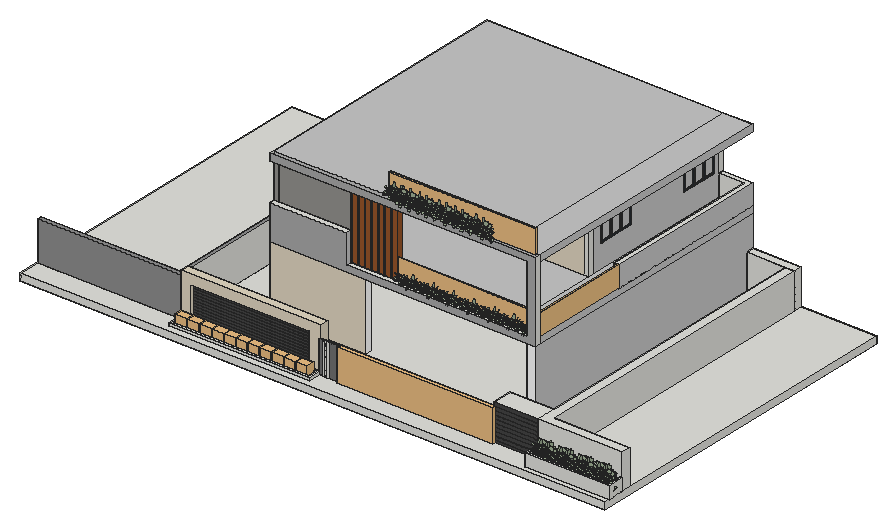
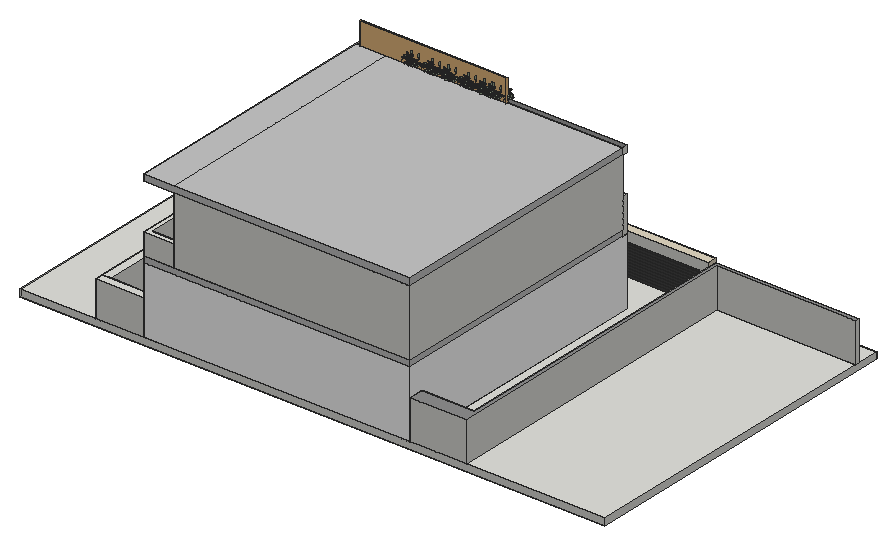
# SketchUp Ruby script. Lengths in inches.
U = 1.inch
M = Sketchup.active_model
def pt(a) = Geom::Point3d.new(a.map { |v| v * U })
def face(e, loops, mat)
  f = e.add_face(loops[0].map { |a| pt(a) })
  loops[1..].each { |l| e.add_face(l.map { |a| pt(a) }).erase! }
  f.material = f.back_material = mat if mat
  f
end
# faces: each face lists its corners as indices into pts; further lists are holes
def faces(e, pts, list, mat = nil) = list.each { |f| face(e, (f[0].is_a?(Array) ? f : [f]).map { |l| l.map { |i| pts[i] } }, mat) }
# xy, xz, yz: faces in a plane at the given z, y or x. An outline is a flat list of corners, or four numbers for a rectangle; further outlines are holes
def ring(l) = l.size == 4 ? [[l[0], l[1]], [l[2], l[1]], [l[2], l[3]], [l[0], l[3]]] : l.each_slice(2).to_a
def flat(e, list, mat, &to3) = list.each { |f| face(e, (f[0].is_a?(Array) ? f : [f]).map { |l| ring(l).map { |u, v| to3.(u, v) } }, mat) }
def xy(e, z, list, mat = nil) = flat(e, list, mat) { |x, y| [x, y, z] }
def xz(e, y, list, mat = nil) = flat(e, list, mat) { |x, z| [x, y, z] }
def yz(e, x, list, mat = nil) = flat(e, list, mat) { |y, z| [x, y, z] }
def lines(e, pts, list) = list.each { |a, b| e.add_line(pt(pts[a]), pt(pts[b])) }
# prism: a flat outline (further loops are holes) pulled along v
def prism(e, loops, v, mat = nil)
  f = face(e, loops, mat); d = Geom::Vector3d.new(v.map { |x| x * U })
  f.pushpull(f.normal.samedirection?(d) ? d.length : -d.length)
end
def box(e, o, s, mat = nil) = prism(e, [[o, [o[0] + s[0], o[1], o[2]], [o[0] + s[0], o[1] + s[1], o[2]], [o[0], o[1] + s[1], o[2]]]], [0, 0, s[2]], mat)
def at(x, y, z, deg = 0) = Geom::Transformation.translation(pt([x, y, z])) * Geom::Transformation.rotation(ORIGIN, Z_AXIS, deg.degrees)
def axes(o, x, y, z) = Geom::Transformation.new([*x, 0, *y, 0, *z, 0, *pt(o).to_a, 1])
def part(name) = M.definitions.add(name)
# library, detail: a bought-in or finely detailed component or shape, given as its bounding box
def library(name, o, s) = part(name).tap { |d| box(d.entities, o, s) }
def detail(e, o, s) = box(e.add_group.entities, o, s)
def put(e, d, t, mat = nil) = e.add_instance(d, t).tap { |i| i.material = mat if mat }
def group(e, t, mat = nil) = e.add_group.tap { |g| g.transformation = t; g.material = mat if mat }.entities
root = M.entities
M.materials.add("Wine2").color = [0, 0, 0]
M.materials["Wine2"].alpha = 0
M.materials.add("[0130_Gainsboro]").color = [39, 45, 50]
M.materials.add("[Color M00]").color = [255, 255, 255]
M.materials.add("[Color M02]").color = [198, 198, 198]
M.materials.add("[Color M03]").color = [170, 170, 170]
M.materials.add("[Color M04]").color = [142, 142, 142]
M.materials.add("[Color M05]").color = [114, 114, 114]
M.materials.add("[Granite Dark Gray]").color = [69, 68, 68]
M.materials.add("[Granite Light Gray]").color = [149, 148, 144]
M.materials.add("[Stone Brushed Khaki]").color = [226, 216, 194]
M.materials.add("[Wood Cherry Original]").color = [152, 86, 42]
M.materials.add("hymenocallis littoralis").color = [156, 172, 146]
c1 = library("Gate",[-51,-3.25,0],[172,7.98,84])
c2 = part("Group\#8")
box(c2.entities,[0,-0.9375,0],[79.125,0.9375,6.23])
c3 = library("Skt_BoxwoodBall_13",[82.21,6.18,-2.42],[14.57,14.83,12.98])
c4 = part("Group\#9")
box(c4.entities,[0,0,0],[5.3125,3.9375,213.9375])
c5 = part("Group\#856")
xy(c5.entities,7.38,[[0,0,5.5,15.91]],"hymenocallis littoralis")
p = [[5.5,28.78,0],[5.5,26.79,3.44],[0,26.79,3.44],[0,28.78,0],[0,23.75,6],[5.5,23.75,6],
  [0,15.91,7.38],[5.5,15.91,7.38]]
faces(c5.entities,p,[[0,1,2,3],[4,2,1,5],[6,4,5,7]],"hymenocallis littoralis")
c6 = part("Group\#854")
xy(c6.entities,7.38,[[0,0,5.5,15.91],[0,15.91,5.5,23.87]],"hymenocallis littoralis")
p = [[5.5,31.07,4.3],[5.5,27.74,6.47],[0,27.74,6.47],[0,31.07,4.3],[0,23.87,7.38],[5.5,23.87,7.38]]
faces(c6.entities,p,[[0,1,2,3],[4,2,1,5]],"hymenocallis littoralis")
c7 = part("Group\#857")
xy(c7.entities,7.38,[[0,0,5.6,15.91]],"hymenocallis littoralis")
p = [[5.6,28.78,0],[5.6,26.79,3.44],[0,26.79,3.44],[0,28.78,0],[0,23.75,6],[5.6,23.75,6],
  [0,15.91,7.38],[5.6,15.91,7.38]]
faces(c7.entities,p,[[0,1,2,3],[4,2,1,5],[6,4,5,7]],"hymenocallis littoralis")
c8 = part("Group\#855")
put(c8.entities,c6,axes([6.09,8.57,-0.52],[0.446,0.85617,0.26089],[-0.18444,-0.19731,0.96283],[0.87582,-0.47754,0.0699]))
put(c8.entities,c6,axes([6.29,7.28,-1.71],[0.37058,0.92707,-0.05667],[-0.32382,0.19004,0.99128],[0.87712,-0.32925,0.34964]))
put(c8.entities,c6,axes([11.04,16.14,-0.7],[1,0,0],[0,0.16628,1.02662],[0,-1.18456,0.19186]))
c9 = part("Group\#860")
put(c9.entities,c5,axes([24.57,32.05,-1.76],[0.9552,-0.22102,-0.19681],[0.4036,0.95545,0.88585],[-0.00568,-0.67859,0.7345]))
put(c9.entities,c5,axes([23.95,29.24,-2.4],[0,1,0],[-0.76041,0,0.64945],[0.64945,0,0.76041]))
put(c9.entities,c5,axes([24.22,24.72,-0.48],[-0.70711,0.70711,0],[-0.32757,-0.32757,0.80237],[0.61237,0.61237,0.5]))
put(c9.entities,c6,axes([20.66,37.22,-0.63],[1.12361,0.03262,0.39091],[-0.43499,0.29739,0.78777],[0.09852,-1.27434,0.37535]))
put(c9.entities,c5,axes([28.75,24.45,-2.4],[-1,0,0],[0,-0.76041,0.64945],[0,0.64945,0.76041]))
put(c9.entities,c7,axes([30.4,30.98,-3.7],[0.65676,-0.72002,0.22414],[0.55667,0.66341,0.5],[-0.50871,-0.20361,0.83652]))
put(c9.entities,c7,axes([32.41,29.61,-3.7],[0.04029,-0.97372,0.22414],[0.85287,0.15038,0.5],[-0.52057,0.17102,0.83652]))
put(c9.entities,c5,axes([31.89,25.85,-1.76],[-0.92056,0.33739,-0.19681],[-0.5186,-0.89824,0.88585],[0.08952,0.67268,0.7345]))
put(c9.entities,c5,axes([25.55,34.78,-0.48],[0.86603,0.5,0],[-0.25,0.43301,0.86603],[0.43301,-0.75,0.5]))
put(c9.entities,c7,axes([20.4,16.9375,-8.07],[-0.70711,0.70711,0],[-0.35754,-0.35754,0.65422],[1.3987,1.3987,1.52882]))
put(c9.entities,c5,axes([32.86,34.14,-0.48],[0.76604,-0.64279,0],[0.32139,0.38302,0.86603],[-0.55667,-0.66341,0.5]))
put(c9.entities,c5,axes([27.15,34.7,-0.1],[0.82472,-0.17528,-0.53769],[0.53769,0.53769,0.64945],[0.17528,-0.82472,0.53769]))
put(c9.entities,c5,axes([33.58,28.77,-2.4],[0,-1,0],[0.76041,0,0.64945],[-0.64945,0,0.76041]))
put(c9.entities,c5,axes([26.43,23.87,-2.81],[-0.75126,0.04415,0.65853],[0.53769,-0.53769,0.64945],[0.38276,0.84199,0.3802]))
put(c9.entities,c5,axes([28.78,23.98,-2.4],[-1,0,0],[0,-0.76041,0.64945],[0,0.64945,0.76041]))
put(c9.entities,c5,axes([25.39,25.38,-2.4],[-0.70711,0.70711,0],[-0.53769,-0.53769,0.64945],[0.45923,0.45923,0.76041]))
put(c9.entities,c5,axes([27.32,21.63,-0.1],[-0.45923,0.70711,-0.53769],[-0.76041,0,0.64945],[0.45923,0.70711,0.53769]))
put(c9.entities,c5,axes([25.17,27.625,-1.76],[0.56416,0.80187,-0.19681],[-0.66673,0.66673,0.80532],[0.62659,-0.26057,0.7345]))
put(c9.entities,c7,axes([27.59,27.04,-3.96],[-0.8993,-0.06127,0.43301],[0.2962,-0.8138,0.5],[0.32175,0.57791,0.75]))
put(c9.entities,c7,axes([26.98,24.5,-3.18],[-0.5,0.86603,0],[-0.75,-0.43301,0.5],[0.43301,0.25,0.86603]))
put(c9.entities,c7,axes([24.55,27.74,-3.7],[0.29517,0.92878,0.22414],[-0.85287,0.15038,0.5],[0.43068,-0.33875,0.83652]))
put(c9.entities,c7,axes([24.26,29.8,-3.18],[0.76604,0.64279,0],[-0.47317,0.5639,0.425],[0.32139,-0.38302,0.86603]))
put(c9.entities,c7,axes([25.98,32.46,-3.18],[1,0,0],[0,0.86603,0.5],[0,-0.5,0.86603]))
put(c9.entities,c5,axes([28.78,33.57,-2.4],[1,0,0],[0,0.76041,0.64945],[0,-0.64945,0.76041]))
put(c9.entities,c8,at(14.99,21.38,2.5))
put(c9.entities,c6,axes([34.63,26.34,-1.46],[-0.70089,-0.70877,0.07994],[0.4756,-0.38088,0.79293],[-0.53156,0.59378,0.60405]))
put(c9.entities,c6,axes([28.14,16.92,1.8125],[-1.19719,0.6912,0],[-0.09607,-0.16641,0.94244],[0.68444,1.18549,0.17613]))
put(c9.entities,c6,axes([31.5625,35.84,0.97],[0.66765,-1.1564,0.35779],[0.04445,0.30732,0.91033],[-1.20828,-0.64496,0.17012]))
put(c9.entities,c6,axes([38.94,22.51,0.89],[-0.97932,-0.67164,-0.05202],[0.27787,-0.41401,0.90999],[-0.85985,0.93577,0.32097]))
put(c9.entities,c6,axes([38.44,21.09,1.98],[-1.02864,-0.54856,0.2395],[0.33481,0.06999,0.88388],[-0.77261,1.08328,0.06417]))
put(c9.entities,c7,axes([35.02,30.51,-1.3],[-0.17365,-0.98481,0],[0.60224,-0.10619,0.79122],[-0.7792,0.13739,0.61153]))
put(c9.entities,c7,axes([29.41,22.33,-1.3],[-0.93969,0.34202,0],[-0.20915,-0.57465,0.79122],[0.27061,0.74351,0.61153]))
put(c9.entities,c6,axes([19.64,36,-1.62],[1.18194,0.09546,0.08234],[-0.14377,0.68823,0.76313],[0.21457,-1.1326,0.62386]))
put(c9.entities,c7,axes([24.25,24.14,-1.3],[-0.34202,0.93969,0],[-0.57465,-0.20915,0.79122],[0.74351,0.27061,0.61153]))
put(c9.entities,c7,axes([25.98,34.61,-1.3],[1,0,0],[0,0.61153,0.79122],[0,-0.79122,0.61153]))
put(c9.entities,c7,axes([31.16,34.41,-1.64],[0.56518,-0.80224,-0.19234],[0.73413,0.34233,0.72935],[-0.47639,-0.50772,0.71782]))
put(c9.entities,c7,axes([40.52,26.84,-5.82],[-0.42262,-0.90631,0],[0.48019,-0.22391,0.68552],[-1.43418,0.66877,1.22305]))
put(c9.entities,c5,axes([29.86,38.42,-1.01],[0.89064,-0.37013,0.26413],[-0.03924,0.63286,1.01918],[-0.45353,-0.76487,0.45748]))
put(c9.entities,c5,axes([29.34,22.4,-0.48],[-0.99619,-0.08716,0],[0.04358,-0.4981,0.86603],[-0.07548,0.86273,0.5]))
c10 = part("Group\#858")
xz(c10.entities,10.07,[[9.07,0,10.07,31.01],[0,31.01,0,45.12,20.13,45.12,20.13,31.01,10.07,31.01,10.07,32.58,9.07,32.58,9.07,31.01]],"hymenocallis littoralis")
yz(c10.entities,10.07,[[0,31.01,20.13,45.12]],"hymenocallis littoralis")
p = [[9.57,9.2,0],[10.07,10.07,0],[10.07,10.07,31.01],[10.07,10.07,32.58],[9.57,9.2,32.58]]
faces(c10.entities,p,[[0,1,2,3,4]],"hymenocallis littoralis")
c11 = part("cây lá nắng")
put(c11.entities,c9,axes([49.26,-2.75,0],[0.63109,0.63109,0],[-0.63109,0.63109,0],[0,0,0.935]))
g1 = group(c11.entities,at(26.6,-8.68,0))
put(g1,c5,axes([-4.72,35.73,-1.65],[0.74231,0.46334,-0.18402],[-0.34827,0.85768,0.82827],[0.42467,-0.43184,0.68675]))
put(g1,c5,axes([-3.34,33.57,-2.24],[-0.63109,0.63109,0],[-0.47989,-0.47989,0.60723],[0.40986,0.40986,0.71098]))
put(g1,c5,axes([-0.3125,30.89,-0.45],[-0.8925,0,0],[0,-0.41345,0.75022],[0,0.77293,0.4675]))
put(g1,c6,axes([-10.79,39.66,-0.59],[0.68852,0.72969,0.3655],[-0.4622,-0.08684,0.73657],[0.86641,-0.74205,0.35095]))
put(g1,c5,axes([2.71,33.57,-2.24],[-0.63109,-0.63109,0],[0.47989,-0.47989,0.60723],[-0.40986,0.40986,0.71098]))
put(g1,c7,axes([-0.37,38.74,-3.46],[0.86887,-0.03992,0.20957],[-0.06737,0.76999,0.4675],[-0.19255,-0.44954,0.78214]))
put(g1,c7,axes([1.76,39.14,-3.46],[0.63993,-0.58908,0.20957],[0.44333,0.63315,0.4675],[-0.43646,-0.2206,0.78214]))
put(g1,c5,axes([3.81,36.4375,-1.65],[-0.79389,-0.36803,-0.18402],[0.23959,-0.89415,0.82827],[-0.36803,0.48102,0.68675]))
put(g1,c5,axes([-5.83,38.07,-0.45],[0.231,0.86209,0],[-0.43104,0.1155,0.80973],[0.74659,-0.20005,0.4675]))
put(g1,c7,axes([2.18,23.5625,-7.55],[-0.8925,0,0],[0,-0.45128,0.6117],[0,1.76542,1.42944]))
put(g1,c5,axes([-0.8125,42.28,-0.45],[0.8891,0.07779,0],[-0.03889,0.44455,0.80973],[0.06737,-0.76999,0.4675]))
put(g1,c5,axes([-4.76,39.03,-0.09],[0.63109,0.40986,-0.50274],[0,0.67866,0.60723],[0.63109,-0.40986,0.50274]))
put(g1,c5,axes([3.03,39.35,-2.24],[0.63109,-0.63109,0],[0.47989,0.47989,0.60723],[-0.40986,-0.40986,0.71098]))
put(g1,c5,axes([1.61,31.74,-2.625],[-0.50198,-0.44625,0.61573],[0.67866,0,0.60723],[-0.28982,0.77293,0.35549]))
put(g1,c5,axes([3.03,33.3,-2.24],[-0.63109,-0.63109,0],[0.47989,-0.47989,0.60723],[-0.40986,0.40986,0.71098]))
put(g1,c5,axes([0.01,32.04,-2.24],[-0.8925,0,0],[0,-0.67866,0.60723],[0,0.57963,0.71098]))
put(g1,c5,axes([3.59,30.89,-0.09],[-0.73607,0.15643,-0.50274],[-0.47989,-0.47989,0.60723],[-0.15643,0.73607,0.50274]))
put(g1,c5,axes([-1.55,33.32,-1.65],[-0.15002,0.86209,-0.18402],[-0.84154,0,0.75297],[0.55988,0.231,0.68675]))
put(g1,c7,axes([0.35,34.48,-3.71],[-0.52887,-0.60621,0.40487],[0.70051,-0.32665,0.4675],[-0.16166,0.56777,0.70125]))
put(g1,c7,axes([2.61,39.13,-1.74],[-0.86209,0.231,0],[-0.23031,-0.85954,0.15531],[0.03162,0.11799,0.91645]))
put(g1,c7,axes([-2.02,33,-3.46],[-0.39986,0.77243,0.20957],[-0.63315,-0.44333,0.4675],[0.48558,0.05802,0.78214]))
put(g1,c7,axes([-3.49,34.12,-2.97],[0.07779,0.8891,0],[-0.65449,0.05726,0.39737],[0.44455,-0.03889,0.80973]))
put(g1,c7,axes([-4.09,36.88,-2.97],[0.63109,0.63109,0],[-0.54654,0.54654,0.4675],[0.31555,-0.31555,0.80973]))
put(g1,c5,axes([-3.02,39.35,-2.24],[0.63109,0.63109,0],[-0.47989,0.47989,0.60723],[0.40986,-0.40986,0.71098]))
put(g1,c8,axes([-4.03,22.95,2.33],[0.63109,0.63109,0],[-0.63109,0.63109,0],[0,0,0.935]))
put(g1,c6,axes([5.24,38.48,-1.37],[0.00497,-0.88963,0.07474],[0.54052,0.05978,0.74139],[-0.71019,0.03927,0.56479]))
put(g1,c6,axes([7.08,28.4375,1.7],[-1.19175,-0.31933,0],[0.04439,-0.16565,0.88118],[-0.31621,1.1801,0.16468]))
put(g1,c6,axes([-2.7,42.54,0.91],[1.15114,-0.30845,0.33454],[-0.1659,0.22199,0.85115],[-0.3555,-1.16957,0.15907]))
put(g1,c6,axes([10.37,38.78,0.83],[-0.19417,-1.04191,-0.04864],[0.43664,-0.08592,0.85084],[-1.1332,0.04791,0.30011]))
put(g1,c6,axes([10.95,37.5625,1.85],[-0.30298,-0.99536,0.22393],[0.16713,0.25547,0.82643],[-1.17124,0.19607,0.06]))
put(g1,c7,axes([2.84,41.36,-1.22],[0.51192,-0.73109,0],[0.44708,0.31305,0.73979],[-0.57846,-0.40504,0.57178]))
put(g1,c7,axes([4.47,32.65,-1.22],[-0.80888,-0.37719,0],[0.23066,-0.49465,0.73979],[-0.29844,0.64,0.57178]))
put(g1,c6,axes([-10.32,35.12,-1.51],[0.68567,0.80616,0.07699],[-0.52507,0.3436,0.71352],[0.85019,-0.57936,0.58331]))
put(g1,c7,axes([0.07,30.54,-1.22],[-0.80888,0.37719,0],[-0.23066,-0.49465,0.73979],[0.29844,0.64,0.57178]))
put(g1,c7,axes([-5.45,38.24,-1.22],[0.63109,0.63109,0],[-0.38593,0.38593,0.73979],[0.49934,-0.49934,0.57178]))
put(g1,c7,axes([-2.05,41.38,-1.53],[0.86296,-0.14961,-0.17984],[0.24726,0.67935,0.68194],[0.01977,-0.62107,0.67116]))
put(g1,c7,axes([8.63,42.51,-5.4375],[0.30525,-0.83868,0],[0.44435,0.16173,0.64096],[-1.32716,-0.48305,1.14356]))
put(g1,c5,axes([-5.4,43.09,-0.94],[0.79566,0.32849,0.24696],[-0.42416,0.37462,0.95293],[0.19648,-0.76892,0.42774]))
put(g1,c5,axes([4.38,32.65,-0.45],[-0.57369,-0.68369,0],[0.34185,-0.28684,0.80973],[-0.5921,0.49683,0.4675]))
put(g1,c7,axes([-2,33.84,-0.15],[-0.24601,0.85793,0],[-0.85539,-0.24528,0.15531],[0.11742,0.03367,0.91645]))
put(g1,c7,axes([0.17,30.83,-4.47],[-0.24601,0.85793,0],[-0.85539,-0.24528,0.15531],[0.11742,0.03367,0.91645]))
put(g1,c7,axes([-1.97,32.18,-4.47],[0.58524,0.67383,0],[-0.67184,0.58351,0.15531],[0.09222,-0.0801,0.91645]))
put(g1,c7,axes([-2,34.71,-4.47],[0.88392,-0.12346,0],[0.12309,0.88131,0.15531],[-0.0169,-0.12098,0.91645]))
put(g1,c7,axes([0.11,36.12,-4.47],[0.37822,-0.8084,0],[0.80601,0.37711,0.15531],[-0.11064,-0.05177,0.91645]))
put(c11.entities,c10,axes([29.71,14.29,6.94],[0.425,0.73612,0],[-0.6771,0.39092,-0.33349],[-0.26859,0.15507,0.72712]))
put(c11.entities,c10,axes([42.0625,26.12,6.94],[0.85,0,0],[0,0.78185,-0.33349],[0,0.33349,0.78185]))
put(c11.entities,c9,axes([7.3125,23.0625,0],[0.8925,0,0],[0,0.8925,0],[0,0,0.935]))
put(c11.entities,c10,axes([24.4375,40.23,2.05],[0.85,0,0],[0,0.85,0],[0,0,0.85]))
c12 = part("Planting 101")
put(c12.entities,c11,axes([21.34,32.96,-4.59],[0,-0.71,0],[-0.71,0,0],[0,0,0.71]))
c13 = part("Facade screen panel")
xy(c13.entities,0,[[0,-0.98,43.07,0],[0,0,43.07,1.4]],"[0130_Gainsboro]")
xy(c13.entities,0.3,[[0.3,-1.43,42.77,-0.98]],"[0130_Gainsboro]")
xy(c13.entities,2.95,[[2.95,-1.43,40.12,-0.63],[2.95,-0.63,40.12,0],[2.95,0,40.12,0.64],[2.95,0.64,40.12,1.4]],"[0130_Gainsboro]")
xy(c13.entities,3.54,[[3.54,-0.63,39.53,0],[3.54,0,39.53,0.64]],"[0130_Gainsboro]")
xy(c13.entities,111.8125,[[3.54,-0.63,39.53,0],[3.54,0,39.53,0.64]],"[0130_Gainsboro]")
xy(c13.entities,112.4,[[2.95,-1.43,40.12,-0.63],[2.95,-0.63,40.12,0],[2.95,0,40.12,0.64],[2.95,0.64,40.12,1.4]],"[0130_Gainsboro]")
xy(c13.entities,115.05,[[0.3,-1.43,42.77,-0.98]],"[0130_Gainsboro]")
xy(c13.entities,115.35,[[0,-0.98,43.07,0],[0,0,43.07,1.4]],"[0130_Gainsboro]")
xz(c13.entities,-1.43,[[[0.3,0.3,42.77,115.05],[2.95,2.95,40.12,112.4]]],"[0130_Gainsboro]")
xz(c13.entities,-0.98,[[[0,0,43.07,115.35],[0.3,0.3,42.77,115.05]]],"[0130_Gainsboro]")
xz(c13.entities,-0.63,[[[2.95,2.95,40.12,112.4],[3.54,3.54,39.53,111.8125]]],"[0130_Gainsboro]")
xz(c13.entities,0,[[3.54,3.54,39.53,111.8125]],"Wine2")
xz(c13.entities,0,[[[0,0,43.07,115.35],[2.95,2.95,40.12,112.4]],[[2.95,2.95,40.12,112.4],[3.54,3.54,39.53,111.8125]]],"[0130_Gainsboro]")
xz(c13.entities,0.64,[[[2.95,2.95,40.12,112.4],[3.54,3.54,39.53,111.8125]]],"[0130_Gainsboro]")
xz(c13.entities,1.4,[[[0,0,43.07,115.35],[2.95,2.95,40.12,112.4]]],"[0130_Gainsboro]")
yz(c13.entities,0,[[-0.98,0,0,115.35],[0,0,1.4,115.35]],"[0130_Gainsboro]")
yz(c13.entities,0.3,[[-1.43,0.3,-0.98,115.05]],"[0130_Gainsboro]")
yz(c13.entities,2.95,[[-1.43,2.95,-0.63,112.4],[-0.63,2.95,0,112.4],[0,2.95,0.64,112.4],[0.64,2.95,1.4,112.4]],"[0130_Gainsboro]")
yz(c13.entities,3.54,[[-0.63,3.54,0,111.8125],[0,3.54,0.64,111.8125]],"[0130_Gainsboro]")
yz(c13.entities,39.53,[[-0.63,3.54,0,111.8125],[0,3.54,0.64,111.8125]],"[0130_Gainsboro]")
yz(c13.entities,40.12,[[-1.43,2.95,-0.63,112.4],[-0.63,2.95,0,112.4],[0,2.95,0.64,112.4],[0.64,2.95,1.4,112.4]],"[0130_Gainsboro]")
yz(c13.entities,42.77,[[-1.43,0.3,-0.98,115.05]],"[0130_Gainsboro]")
yz(c13.entities,43.07,[[-0.98,0,0,115.35],[0,0,1.4,115.35]],"[0130_Gainsboro]")
c14 = part("Facade screen assembly")
put(c14.entities,c13,axes([90.57,1.43,0],[1.05148,0,0],[0,1,0],[0,0,1]))
put(c14.entities,c13,axes([0,1.43,0],[1.05148,0,0],[0,1,0],[0,0,1]))
put(c14.entities,c13,axes([45.29,1.43,0],[1.05148,0,0],[0,1,0],[0,0,1]))
c15 = part("Group\#1")
prism(c15.entities,[[[0,0,12],[425.4375,0,12],[480,0,12],[480,0,0],[0,0,0]]],[0,-480,0])
c16 = library("Wagner Glass Railing",[9.08,102.375,1.53],[2.51,145.5,42.05])
c17 = part("Group\#2")
box(c17.entities,[0,0,0],[10.47,9,122.5625])
xy(root,-144,[[510.07,35.9375,546.61,39.0625]])
xy(root,-132,[[907.13,15.54,1048.98,33.86],[907.13,33.86,1048.98,39.0625],[0,39.0625,0,46.74,249.6875,46.74,249.6875,611.75,352.1875,611.75,352.1875,584.91,257.75,584.91,257.75,39.0625],[257.75,39.0625,275.38,56],[489.36,39.0625,486.83,56,510.07,56,510.07,39.0625],
  [822.8,39.0625,822.8,75.52,901.93,75.52,901.93,596.5625,918.875,596.5625,918.875,55.89,1054.1875,55.89,1054.1875,39.0625],[352.1875,121.8125,525.92,121.8125,525.92,132.95,374.05,132.95,374.05,303.74,529.67,303.74,529.67,587.11,815.55,587.11,815.55,121.8125,832.1875,121.8125,832.1875,611.75,352.1875,611.75],[832.1875,596.5625,918.875,611.75]])
xy(root,-131.6875,[[262.47,18.27,505.61,34.35]])
xy(root,-127.875,[[[257.75,13.5625,510.32,39.0625],[262.47,18.27,505.61,34.35]]])
xy(root,-110.4375,[[901.93,10.34,901.93,39.0625,907.13,39.0625,907.13,15.54,1048.98,15.54,1048.98,39.0625,1054.1875,39.0625,1054.1875,10.34]])
xy(root,-74.28,[[510.07,35.9375,546.61,39.0625]],"[Color M05]")
xy(root,-71.16,[[275.38,39.0625,275.38,56,486.83,56,489.36,39.0625]],"[Stone Brushed Khaki]")
xy(root,-68.0625,[[822.8,39.0625,901.93,75.52],[901.93,39.0625,1054.1875,39.0625,1054.1875,55.89,918.875,55.89,918.875,596.5625,901.93,596.5625],[832.1875,596.5625,918.875,611.75]])
xy(root,-60.875,[[0,39.0625,257.75,39.0625,257.75,584.91,352.1875,584.91,352.1875,611.75,249.6875,611.75,249.6875,46.74,0,46.74]],"[Color M04]")
xy(root,-54.1875,[[257.75,39.0625,510.07,56]],"[Stone Brushed Khaki]")
xy(root,-12,[[352.1875,121.8125,525.92,131.75],[525.92,121.8125,815.55,131.75],[815.55,121.8125,832.1875,131.75],[525.92,143.67,815.55,171.7],[815.55,143.67,832.1875,171.7]])
xy(root,-12,[[352.1875,131.75,352.1875,143.67,374.05,143.67,374.05,132.95,525.92,132.95,525.92,131.75],[815.55,131.75,832.1875,143.67],[374.05,132.95,525.92,143.67],[374.05,143.67,525.92,171.7],[352.1875,171.7,352.1875,611.75,832.1875,611.75,832.1875,171.7,815.55,171.7,815.55,587.11,529.67,587.11,529.67,303.74,374.05,303.74,374.05,171.7]],"[Color M00]")
xy(root,0,[[491.36,121.8125,815.21,131.75],[[352.1875,131.75,361.1875,131.75,361.1875,308.68,777.625,308.68,777.625,611.75,352.1875,611.75],[361.1875,317.68,768.625,602.75]],[491.36,131.75,492.47,140.75],[502.94,131.75,823.1875,131.75,823.1875,140.75,777.625,140.75,777.625,308.68,768.625,308.68,768.625,140.75,502.94,140.75],[823.1875,131.75,832.1875,308.68],
  [361.1875,140.75,768.625,308.68],[777.625,140.75,823.1875,308.68],[777.625,308.68,823.1875,317.68],[361.1875,317.68,768.625,602.75],[777.625,317.68,823.1875,602.75]])
xy(root,38.23,[[823.1875,308.68,832.1875,308.68,832.1875,611.75,777.625,611.75,777.625,602.75,823.1875,602.75]])
xy(root,52.4375,[[352.1875,121.8125,491.36,131.75]])
xy(root,120,[[352.1875,121.8125,361.1875,131.75],[361.1875,121.8125,815.21,131.75],[[352.1875,131.75,361.1875,131.75,361.1875,308.68,777.625,308.68,777.625,611.75,352.1875,611.75],[361.1875,317.68,768.625,602.75]],[361.1875,131.75,491.36,140.75]])
xz(root,10.34,[[901.93,-132,1054.1875,-110.4375]])
xz(root,13.5625,[[257.75,-132,510.32,-127.875]])
xz(root,15.54,[[907.13,-132,1048.98,-110.4375]])
xz(root,18.27,[[262.47,-131.6875,505.61,-127.875]])
xz(root,34.35,[[262.47,-131.6875,275.38,-127.875],[275.38,-131.6875,489.36,-127.875],[489.36,-131.6875,505.61,-127.875]])
xz(root,35.9375,[[513.3,-132,515.14,-74.28],[516.66,-132,518.82,-74.28],[520.56,-132,522.85,-74.28],[524.61,-132,527.05,-74.28]])
xz(root,35.9375,[[510.07,-144,546.61,-144,546.61,-74.28,527.05,-74.28,527.05,-132,524.61,-132,524.61,-74.28,522.85,-74.28,522.85,-132,520.56,-132,520.56,-74.28,518.82,-74.28,518.82,-132,516.66,-132,516.66,-74.28,515.14,-74.28,515.14,-132,513.3,-132,513.3,-74.28,510.07,-74.28]],"[Color M05]")
xz(root,39.0625,[[510.07,-144,510.07,-132,510.32,-132,510.32,-127.875,510.07,-127.875,510.07,-74.28,546.61,-74.28,546.61,-144],[257.75,-132,275.38,-127.875],[275.38,-132,489.36,-127.875],[489.36,-132,510.07,-127.875],[510.07,-132,510.32,-127.875],
  [822.8,-132,901.93,-74.29],[901.93,-132,907.13,-110.4375],[907.13,-132,1048.98,-132,1048.98,-110.4375,1054.1875,-110.4375,1054.1875,-68.0625,901.93,-68.0625,901.93,-110.4375,907.13,-110.4375],[1048.98,-132,1054.1875,-110.4375]])
xz(root,39.0625,[[0,-132,257.75,-60.875]],"[Color M04]")
xz(root,39.0625,[[257.75,-127.875,275.38,-127.875,275.38,-71.16,489.36,-71.16,489.36,-127.875,510.07,-127.875,510.07,-54.1875,257.75,-54.1875]],"[Stone Brushed Khaki]")
xz(root,46.74,[[0,-132,249.6875,-60.875]])
xz(root,55.89,[[918.875,-132,1054.1875,-68.0625]])
xz(root,56,[[257.75,-132,257.75,-54.1875,510.07,-54.1875,510.07,-132,486.83,-132,486.83,-71.16,275.38,-71.16,275.38,-132]])
xz(root,75.52,[[822.8,-132,901.93,-68.0625]])
xz(root,121.8125,[[815.55,-132,832.1875,-12]],"[Color M00]")
xz(root,121.8125,[[352.1875,-12,832.1875,-12,832.1875,132,352.1875,132,352.1875,120,815.21,120,815.21,0,491.36,0,491.36,52.4375,352.1875,52.4375]],"[Color M03]")
xz(root,121.8125,[[352.1875,-132,525.92,-12]],"[Stone Brushed Khaki]")
xz(root,131.75,[[352.1875,-12,352.1875,0,361.1875,0,361.1875,52.4375,491.36,52.4375,491.36,0,832.1875,0,832.1875,-12],[352.1875,0,361.1875,52.4375],[815.21,0,832.1875,120]])
xz(root,131.75,[[352.1875,52.4375,361.1875,120],[361.1875,52.4375,491.36,120]],"[Granite Light Gray]")
xz(root,132.95,[[374.05,-132,525.92,-12]],"[Color M00]")
xz(root,140.75,[[361.1875,0,491.36,120]])
xz(root,303.74,[[374.05,-132,529.67,-12]],"[Color M05]")
xz(root,308.68,[[768.625,0,777.625,120],[823.1875,0,832.1875,38.23]])
xz(root,308.68,[[361.1875,0,768.625,120]],"[Stone Brushed Khaki]")
xz(root,317.68,[[361.1875,0,768.625,120]])
xz(root,584.91,[[257.75,-132,352.1875,-60.875]])
xz(root,587.11,[[529.67,-132,815.55,-12]],"[Color M00]")
xz(root,596.5625,[[832.1875,-132,901.93,-68.0625],[901.93,-132,918.875,-68.0625]])
xz(root,602.75,[[361.1875,0,768.625,120],[777.625,0,823.1875,38.23]])
xz(root,611.75,[[249.6875,-132,352.1875,-60.875],[832.1875,-132,918.875,-68.0625],[352.1875,0,777.625,120],[777.625,0,832.1875,38.23]])
xz(root,611.75,[[352.1875,-132,832.1875,-12]],"[Color M00]")
yz(root,0,[[39.0625,-132,46.74,-60.875]])
yz(root,249.6875,[[46.74,-132,611.75,-60.875]])
yz(root,257.75,[[13.5625,-132,39.0625,-127.875],[39.0625,-132,56,-60.875],[56,-132,584.91,-60.875]])
yz(root,257.75,[[39.0625,-60.875,56,-54.1875]],"[Stone Brushed Khaki]")
yz(root,262.47,[[18.27,-131.6875,34.35,-127.875]])
yz(root,275.38,[[39.0625,-132,56,-71.16]],"[Stone Brushed Khaki]")
yz(root,352.1875,[[584.91,-132,611.75,-60.875],[121.8125,-12,131.75,52.4375],[131.75,0,611.75,120],[121.8125,120,131.75,132]])
yz(root,352.1875,[[121.8125,-132,584.91,-132,584.91,-60.875,611.75,-60.875,611.75,-12,121.8125,-12]],"[Color M00]")
yz(root,361.1875,[[131.75,0,140.75,120],[317.68,0,602.75,120]])
yz(root,361.1875,[[140.75,0,308.68,120]],"[Color M02]")
yz(root,374.05,[[132.95,-132,303.74,-12]],"[Color M00]")
yz(root,491.36,[[131.75,0,140.75,120]])
yz(root,491.36,[[121.8125,0,131.75,52.4375]],"[Color M02]")
yz(root,505.61,[[18.27,-131.6875,34.35,-127.875]])
yz(root,510.07,[[35.9375,-144,39.0625,-74.28]])
yz(root,510.07,[[39.0625,-132,56,-54.1875]],"[Stone Brushed Khaki]")
yz(root,510.32,[[13.5625,-132,39.0625,-127.875]])
yz(root,525.92,[[121.8125,-132,132.95,-12]],"[Color M00]")
yz(root,529.67,[[303.74,-132,587.11,-12]],"[Stone Brushed Khaki]")
yz(root,546.61,[[35.9375,-144,39.0625,-74.28]])
yz(root,768.625,[[317.68,0,602.75,120]])
yz(root,777.625,[[308.68,0,317.68,120],[602.75,0,611.75,38.23],[602.75,38.23,611.75,120]])
yz(root,777.625,[[317.68,0,602.75,120]],"[Color M02]")
yz(root,815.21,[[121.8125,0,131.75,120]])
yz(root,815.55,[[121.8125,-132,587.11,-12]],"[Color M00]")
yz(root,822.8,[[39.0625,-132,75.52,-68.0625]])
yz(root,823.1875,[[308.68,0,602.75,38.23]])
yz(root,832.1875,[[596.5625,-132,611.75,-68.0625],[121.8125,-12,131.75,132]])
yz(root,832.1875,[[121.8125,-132,121.8125,-12,611.75,-12,611.75,-68.0625,596.5625,-68.0625,596.5625,-132],[308.68,0,611.75,38.23]],"[Color M02]")
yz(root,901.93,[[10.34,-132,39.0625,-110.4375],[75.52,-132,596.5625,-68.0625]])
yz(root,907.13,[[15.54,-132,33.86,-110.4375],[33.86,-132,39.0625,-110.4375]])
yz(root,918.875,[[55.89,-132,596.5625,-68.0625],[596.5625,-132,611.75,-68.0625]])
yz(root,1048.98,[[15.54,-132,33.86,-110.4375],[33.86,-132,39.0625,-110.4375]])
yz(root,1054.1875,[[10.34,-132,39.0625,-110.4375],[39.0625,-132,55.89,-68.0625]])
p = [[489.36,39.0625,-71.16],[486.83,56,-71.16],[486.83,56,-132],[489.36,39.0625,-132],[489.36,39.0625,-127.875]]
faces(root,p,[[0,1,2,3,4]],"[Stone Brushed Khaki]")
g2 = group(root,at(352.1875,611.75,-144))
box(g2,[-352.1875,-611.75,0],[1054.1875,611.75,12])
put(root,c1,axes([628.11,35.9375,-144],[1.63,0,0],[0,1,0],[0,0,0.83]))
put(root,c2,at(822.8,39.0625,-142.23),"[Granite Dark Gray]")
put(root,c3,axes([208.55,15.05,-131.6],[1.46,0,0],[0,1,0],[0,0,1.48]))
put(root,c3,axes([230.11,15.05,-131.6],[1.46,0,0],[0,1,0],[0,0,1.48]))
put(root,c3,axes([250.98,15.05,-131.6],[1.46,0,0],[0,1,0],[0,0,1.48]))
put(root,c3,axes([272.36,15.05,-131.6],[1.46,0,0],[0,1,0],[0,0,1.48]))
put(root,c3,axes([294.11,15.05,-131.6],[1.46,0,0],[0,1,0],[0,0,1.48]))
put(root,c3,axes([316.48,15.05,-131.6],[1.46,0,0],[0,1,0],[0,0,1.48]))
put(root,c3,axes([337.55,15.05,-131.6],[1.46,0,0],[0,1,0],[0,0,1.48]))
put(root,c3,axes([359.11,15.05,-131.6],[1.46,0,0],[0,1,0],[0,0,1.48]))
put(root,c2,at(822.8,39.0625,-135.1),"[Granite Dark Gray]")
put(root,c3,axes([142.28,13.91,-130.83],[1.46,0,0],[0,1,0],[0,0,1.48]))
put(root,c3,axes([164.97,13.91,-130.83],[1.46,0,0],[0,1,0],[0,0,1.48]))
put(root,c3,axes([187.28,13.91,-130.83],[1.46,0,0],[0,1,0],[0,0,1.48]))
put(root,c4,axes([275.38,45.15,-132],[0,1,0],[0,0,1],[1,0,0]),"[Granite Dark Gray]")
put(root,c2,at(822.8,39.0625,-128.16),"[Granite Dark Gray]")
put(root,c4,axes([275.38,45.15,-127.0625],[0,1,0],[0,0,1],[1,0,0]),"[Granite Dark Gray]")
put(root,c12,axes([919.06,24.34,-116.2],[0,-0.53939,0],[1,0,0],[0,0,1]))
put(root,c12,axes([955.25,24.34,-116.2],[0,-0.53939,0],[1,0,0],[0,0,1]))
put(root,c12,axes([990.75,24.34,-116.2],[0,-0.53939,0],[1,0,0],[0,0,1]))
put(root,c12,axes([1023.62,24.34,-116.2],[0,-0.53939,0],[1,0,0],[0,0,1]))
put(root,c14,axes([639.37,575.11,-123.22],[0.72,0,0],[0,0.72,0],[0,0,0.72]))
put(root,c4,axes([275.38,45.15,-122.1875],[0,1,0],[0,0,1],[1,0,0]),"[Granite Dark Gray]")
put(root,c2,at(822.8,39.0625,-121.16),"[Granite Dark Gray]")
put(root,c4,axes([275.38,45.15,-117.1875],[0,1,0],[0,0,1],[1,0,0]),"[Granite Dark Gray]")
put(root,c2,at(822.8,39.0625,-114.35),"[Granite Dark Gray]")
put(root,c4,axes([275.38,45.15,-112.4375],[0,1,0],[0,0,1],[1,0,0]),"[Granite Dark Gray]")
put(root,c2,at(822.8,39.0625,-107.6),"[Granite Dark Gray]")
put(root,c4,axes([275.38,45.15,-107.5],[0,1,0],[0,0,1],[1,0,0]),"[Granite Dark Gray]")
put(root,c4,axes([275.38,45.15,-102.8125],[0,1,0],[0,0,1],[1,0,0]),"[Granite Dark Gray]")
put(root,c2,at(822.8,39.0625,-100.98),"[Granite Dark Gray]")
put(root,c4,axes([275.38,45.15,-97.9375],[0,1,0],[0,0,1],[1,0,0]),"[Granite Dark Gray]")
put(root,c2,at(822.8,39.0625,-94.29),"[Granite Dark Gray]")
put(root,c4,axes([275.38,45.15,-93],[0,1,0],[0,0,1],[1,0,0]),"[Granite Dark Gray]")
put(root,c4,axes([275.38,45.15,-87.9375],[0,1,0],[0,0,1],[1,0,0]),"[Granite Dark Gray]")
put(root,c2,at(822.8,39.0625,-87.66),"[Granite Dark Gray]")
put(root,c4,axes([275.38,45.15,-83.4375],[0,1,0],[0,0,1],[1,0,0]),"[Granite Dark Gray]")
put(root,c2,at(822.8,39.0625,-81.04),"[Granite Dark Gray]")
put(root,c4,axes([275.38,45.15,-78.64],[0,1,0],[0,0,1],[1,0,0]),"[Granite Dark Gray]")
put(root,c2,at(822.8,39.0625,-74.29),"[Granite Dark Gray]")
put(root,c4,axes([275.38,45.15,-73.64],[0,1,0],[0,0,1],[1,0,0]),"[Granite Dark Gray]")
put(root,c12,axes([585.69,131.92,-4.12],[0,-0.53939,0],[1,0,0],[0,0,1]))
put(root,c12,axes([622.88,131.92,-4.12],[0,-0.53939,0],[1,0,0],[0,0,1]))
put(root,c12,axes([658.57,131.92,-4.12],[0,-0.53939,0],[1,0,0],[0,0,1]))
put(root,c12,axes([695.69,131.92,-4.12],[0,-0.53939,0],[1,0,0],[0,0,1]))
put(root,c12,axes([732.69,131.92,-4.12],[0,-0.53939,0],[1,0,0],[0,0,1]))
put(root,c12,axes([767.44,131.92,-4.12],[0,-0.53939,0],[1,0,0],[0,0,1]))
put(root,c12,axes([795.19,131.92,-4.12],[0,-0.53939,0],[1,0,0],[0,0,1]))
put(root,c15,at(352.1875,611.75,-12),"[Color M02]")
put(root,c16,axes([405.87,143.25,-5.66],[0,-1,0],[1.65309,0,0],[0,0,1]))
put(root,c17,at(492.47,131.75,0),"[Wood Cherry Original]")
put(root,c17,at(504.47,131.75,0),"[Wood Cherry Original]")
put(root,c17,at(516.47,131.75,0),"[Wood Cherry Original]")
put(root,c17,at(540.47,131.75,0),"[Wood Cherry Original]")
put(root,c17,at(552.47,131.75,0),"[Wood Cherry Original]")
put(root,c17,at(564.47,131.75,0),"[Wood Cherry Original]")
put(root,c17,at(528.47,131.75,0),"[Wood Cherry Original]")
put(root,c16,axes([821.34,7.26,-0.46],[1,0,0],[0,1.21599,0],[0,0,0.897]))
put(root,c14,axes([778.33,336.97,42.79],[0,0.4896,0],[-0.4896,0,0],[0,0,0.4896]))
put(root,c14,axes([778.33,523.22,42.79],[0,0.4896,0],[-0.4896,0,0],[0,0,0.4896]))
put(root,c15,at(352.1875,611.75,120),"[Color M02]")
put(root,c12,axes([720.97,124.83,133.7],[0,-0.53939,0],[1,0,0],[0,0,1]))
put(root,c12,axes([684.1,124.83,133.7],[0,-0.53939,0],[1,0,0],[0,0,1]))
put(root,c12,axes([654.11,124.83,133.7],[0,-0.53939,0],[1,0,0],[0,0,1]))
put(root,c12,axes([619.36,124.83,133.7],[0,-0.53939,0],[1,0,0],[0,0,1]))
put(root,c12,axes([589.67,124.83,133.7],[0,-0.53939,0],[1,0,0],[0,0,1]))
put(root,c12,axes([573.36,124.83,133.7],[0,-0.53939,0],[1,0,0],[0,0,1]))
put(root,c16,axes([374.83,142.375,128.15],[0,-1,0],[1.81443,0,0],[0,0,1]))
